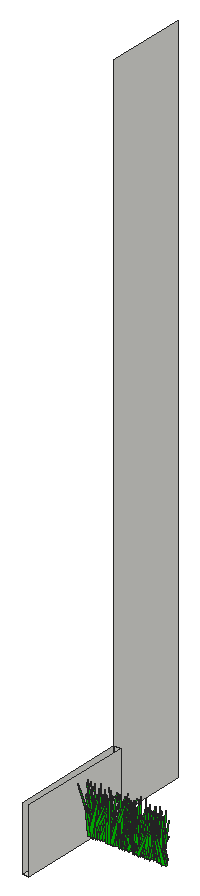
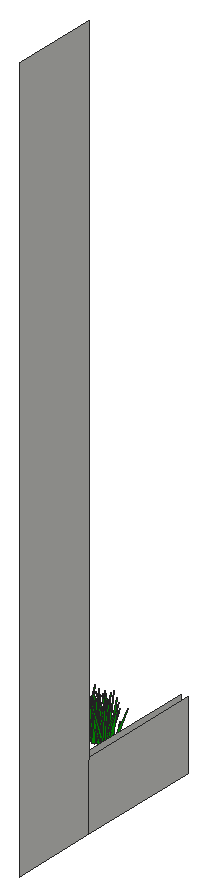
# SketchUp Ruby script. Lengths in inches.
U = 1.inch
M = Sketchup.active_model
def pt(a) = Geom::Point3d.new(a.map { |v| v * U })
def face(e, loops, mat)
  f = e.add_face(loops[0].map { |a| pt(a) })
  loops[1..].each { |l| e.add_face(l.map { |a| pt(a) }).erase! }
  f.material = f.back_material = mat if mat
  f
end
# faces: each face lists its corners as indices into pts; further lists are holes
def faces(e, pts, list, mat = nil) = list.each { |f| face(e, (f[0].is_a?(Array) ? f : [f]).map { |l| l.map { |i| pts[i] } }, mat) }
# xy, xz, yz: faces in a plane at the given z, y or x. An outline is a flat list of corners, or four numbers for a rectangle; further outlines are holes
def ring(l) = l.size == 4 ? [[l[0], l[1]], [l[2], l[1]], [l[2], l[3]], [l[0], l[3]]] : l.each_slice(2).to_a
def flat(e, list, mat, &to3) = list.each { |f| face(e, (f[0].is_a?(Array) ? f : [f]).map { |l| ring(l).map { |u, v| to3.(u, v) } }, mat) }
def xy(e, z, list, mat = nil) = flat(e, list, mat) { |x, y| [x, y, z] }
def xz(e, y, list, mat = nil) = flat(e, list, mat) { |x, z| [x, y, z] }
def yz(e, x, list, mat = nil) = flat(e, list, mat) { |y, z| [x, y, z] }
def lines(e, pts, list) = list.each { |a, b| e.add_line(pt(pts[a]), pt(pts[b])) }
# prism: a flat outline (further loops are holes) pulled along v
def prism(e, loops, v, mat = nil)
  f = face(e, loops, mat); d = Geom::Vector3d.new(v.map { |x| x * U })
  f.pushpull(f.normal.samedirection?(d) ? d.length : -d.length)
end
def box(e, o, s, mat = nil) = prism(e, [[o, [o[0] + s[0], o[1], o[2]], [o[0] + s[0], o[1] + s[1], o[2]], [o[0], o[1] + s[1], o[2]]]], [0, 0, s[2]], mat)
def at(x, y, z, deg = 0) = Geom::Transformation.translation(pt([x, y, z])) * Geom::Transformation.rotation(ORIGIN, Z_AXIS, deg.degrees)
def axes(o, x, y, z) = Geom::Transformation.new([*x, 0, *y, 0, *z, 0, *pt(o).to_a, 1])
def part(name) = M.definitions.add(name)
# library, detail: a bought-in or finely detailed component or shape, given as its bounding box
def library(name, o, s) = part(name).tap { |d| box(d.entities, o, s) }
def detail(e, o, s) = box(e.add_group.entities, o, s)
def put(e, d, t, mat = nil) = e.add_instance(d, t).tap { |i| i.material = mat if mat }
def group(e, t, mat = nil) = e.add_group.tap { |g| g.transformation = t; g.material = mat if mat }.entities
root = M.entities
M.materials.add("[Color G06]").color = [0, 204, 0]
c1 = part("fur_instance\#9")
p = [[0.8125,0,1.79],[0.67,-0.02,1.48],[0,-0.11,0],[0,0.11,0]]
faces(c1.entities,p,[[0,1,2,3]])
xy(root,-6,[[0,8.54,2.44,50.4375]])
xz(root,50.4375,[[0,-6,2.44,17.375]])
yz(root,0,[[8.54,-6,50.4375,17.375],[50.4375,-6,79.8125,242.375]])
yz(root,2.44,[[8.54,-6,50.4375,17.375]])
put(root,c1,axes([12.85,23.35,4.28],[1.6552,-0.74425,1.711],[-5.30221,-0.17956,2.48509],[1.29737,0.21567,7.97338]),"[Color G06]")
put(root,c1,axes([30.55,23.19,4.28],[2.41886,0.55777,0.72324],[3.70499,-0.277,-3.1391],[1.58316,-0.20395,6.24128]),"[Color G06]")
put(root,c1,axes([19.93,23.08,4.28],[3.91287,0.46148,2.2279],[3.1944,-0.58296,1.33945],[-1.72336,-0.03279,7.54123]),"[Color G06]")
put(root,c1,axes([25.93,23.0625,4.28],[5.73991,0.1518,2.08448],[0.76165,-0.80795,2.07407],[-1.5969,0.16027,8.48172]),"[Color G06]")
put(root,c1,axes([28.37,23.59,4.28],[-5.0246,-0.07076,3.70183],[0.48716,0.7269,3.07314],[2.48091,-0.28604,6.89387]),"[Color G06]")
put(root,c1,axes([12.63,23.18,4.28],[-0.11389,0.42663,0.38922],[2.96453,0.00581,1.20582],[-0.79981,-0.03921,4.41401]),"[Color G06]")
put(root,c1,axes([28.8,23.47,4.28],[-3.12756,-0.15217,0.72398],[-0.95592,0.43262,1.2217],[0.71538,-0.0872,4.79764]),"[Color G06]")
put(root,c1,axes([34.63,23.32,4.28],[-0.5319,-0.36164,2.3884],[-2.75252,0.15397,1.30884],[1.30505,0.17735,3.73398]),"[Color G06]")
put(root,c1,axes([33.33,23.2,4.28],[1.33106,0.36919,0.76233],[2.20259,-0.19464,2.23785],[-1.55515,0.04033,3.822]),"[Color G06]")
put(root,c1,axes([28.54,23.35,4.28],[-2.39958,-0.23418,0.91403],[-1.7872,0.31366,-1.24928],[-0.0094,0.14442,4.19532]),"[Color G06]")
put(root,c1,axes([13.41,23.41,4.28],[1.72403,-0.72016,2.8767],[-4.93971,-0.07717,4.39354],[2.4445,0.35197,6.84936]),"[Color G06]")
put(root,c1,axes([30.17,23.48,4.28],[2.8945,0.2824,1.41715],[2.22418,-0.38591,-1.31377],[-0.23073,-0.1774,5.11367]),"[Color G06]")
put(root,c1,axes([25.15,23.2,4.28],[4.85525,0.25985,0.85646],[1.64604,-0.6613,2.20422],[-1.04468,0.16571,7.45353]),"[Color G06]")
put(root,c1,axes([23.65,23.29,4.28],[2.63832,0.09566,1.76868],[0.13664,-0.37516,1.87571],[-1.36103,0.14778,3.61684]),"[Color G06]")
put(root,c1,axes([39.7,23.3,4.28],[-1.60341,0.64726,0.46513],[4.41157,0.19699,2.48074],[-1.47638,-0.11433,6.90756]),"[Color G06]")
put(root,c1,axes([14.0625,23.39,4.28],[2.53929,-0.11197,1.32679],[-1.06003,-0.3452,1.18522],[-0.55601,0.14677,3.79981]),"[Color G06]")
put(root,c1,axes([30.79,23.91,4.28],[4.96251,-0.35133,2.15293],[-1.47007,-0.64737,-4.56652],[-2.50232,-0.31642,6.95237]),"[Color G06]")
put(root,c1,axes([20.78,23.25,4.28],[1.34252,0.72283,0.0164],[5.00506,-0.18035,-2.08662],[1.34888,-0.05024,7.72612]),"[Color G06]")
put(root,c1,axes([29.4375,23.32,4.28],[-1.28557,0.59423,1.27715],[4.16234,0.20409,-1.54961],[1.25078,-0.06842,6.46945]),"[Color G06]")
put(root,c1,axes([32.22,23.53,4.28],[-5.11111,0.1924,0.36372],[1.40056,0.7051,1.11518],[0.03793,-0.10931,7.8334]),"[Color G06]")
put(root,c1,axes([29.77,23.65,4.28],[-1.3987,-0.81448,2.72919],[-5.9965,0.23455,1.17629],[1.22159,0.21879,8.89902]),"[Color G06]")
put(root,c1,axes([20.625,23.68,4.28],[2.09428,-0.78657,0.87313],[-5.32436,-0.24284,3.39616],[1.95198,0.18152,8.32683]),"[Color G06]")
put(root,c1,axes([18.4,23.57,4.28],[2.99741,0.29568,0.585],[2.13228,-0.39259,-1.61022],[0.32024,-0.15348,5.24587]),"[Color G06]")
put(root,c1,axes([24.57,23.56,4.28],[-2.31586,-0.36535,0.62633],[-2.55714,0.28662,-1.91374],[-0.708,0.15984,4.86328]),"[Color G06]")
put(root,c1,axes([33,23.48,4.28],[4.91073,-0.40144,3.20689],[-3.31936,-0.70084,1.27585],[-1.36875,0.25935,8.41144]),"[Color G06]")
put(root,c1,axes([21.69,23.48,4.28],[2.25116,0.46724,2.42365],[3.3843,-0.36695,1.10474],[-1.55026,-0.12258,5.93111]),"[Color G06]")
put(root,c1,axes([15.98,23.37,4.28],[2.98241,0.27292,0.8081],[1.72101,-0.41087,1.75207],[-1.07746,0.09916,5.0354]),"[Color G06]")
put(root,c1,axes([33.29,23.39,4.28],[-0.61548,0.71183,1.08792],[4.98232,0.05576,2.10506],[-1.32848,-0.12066,7.39074]),"[Color G06]")
put(root,c1,axes([28.35,23.79,4.28],[-2.2351,-0.42611,1.57336],[-2.51511,0.3414,2.64062],[2.02982,-0.04618,5.00443]),"[Color G06]")
put(root,c1,axes([38.11,23.43,4.28],[-0.76903,0.72137,2.0022],[5.23961,0.13887,-1.25216],[1.04989,-0.16466,7.71563]),"[Color G06]")
put(root,c1,axes([13.86,23.61,4.28],[2.71632,-0.46654,0.25104],[-3.00104,-0.32551,3.04278],[1.48844,0.1951,5.67683]),"[Color G06]")
put(root,c1,axes([14.85,23.34,4.28],[-3.57418,0.15931,1.87457],[0.45728,0.48323,-2.77015],[1.6338,0.21327,4.87623]),"[Color G06]")
put(root,c1,axes([23,23.73,4.28],[5.38084,0.01238,0.72227],[0.17983,-0.73926,-1.53704],[-0.45725,-0.14506,7.89493]),"[Color G06]")
put(root,c1,axes([16.29,23.63,4.28],[2.30947,0.32228,0.62027],[2.26105,-0.28332,-1.89459],[0.63352,-0.16368,4.50067]),"[Color G06]")
put(root,c1,axes([13.13,23.65,4.28],[1.72877,-0.45008,0.49631],[-2.65707,-0.16626,3.3536],[1.86221,0.1806,4.32429]),"[Color G06]")
put(root,c1,axes([19.2,23.38,4.28],[0.80978,0.69046,0.59357],[4.8898,-0.12068,1.22501],[-0.87466,-0.03542,7.39796]),"[Color G06]")
put(root,c1,axes([18.43,23.79,4.28],[4.45416,-0.00649,0.14759],[-0.01839,-0.59853,-1.78589],[-0.10762,-0.16652,6.41343]),"[Color G06]")
put(root,c1,axes([28.8125,23.49,4.28],[-2.35811,0.38989,1.71965],[2.55865,0.36574,-1.68843],[1.61083,-0.01018,5.19933]),"[Color G06]")
put(root,c1,axes([34.9,23.99,4.28],[3.97939,-0.66126,1.5906],[-4.29861,-0.56838,-3.12205],[-2.26762,-0.08298,8.70959]),"[Color G06]")
put(root,c1,axes([40.57,23.5625,4.28],[-4.2997,-0.26227,1.133],[-2.02384,0.57059,-1.9831],[0.12754,0.21235,6.72796]),"[Color G06]")
put(root,c1,axes([30.6875,23.8,4.28],[1.06399,-0.58128,0.38184],[-3.56039,-0.10703,3.44347],[2.18298,0.10875,5.43011]),"[Color G06]")
put(root,c1,axes([15.04,23.89,4.28],[2.29731,-0.39502,0.33746],[-2.68324,-0.31485,-1.53547],[-0.93594,-0.06694,5.23035]),"[Color G06]")
put(root,c1,axes([26.5,23.68,4.28],[2.69023,-0.58504,0.88466],[-3.7722,-0.28619,3.88244],[1.92943,0.2562,6.35698]),"[Color G06]")
put(root,c1,axes([14.56,23.65,4.28],[-0.73248,0.41655,1.23313],[2.91888,0.05301,1.81602],[-1.04133,-0.14443,4.22295]),"[Color G06]")
put(root,c1,axes([29.15,23.39,4.28],[-5.18337,0.20223,2.51266],[0.67358,0.71057,-3.46575],[2.11562,0.26923,7.25958]),"[Color G06]")
put(root,c1,axes([27.24,24.04,4.28],[4.6175,-0.53623,1.55109],[-3.45439,-0.64944,-2.82084],[-1.98282,-0.11731,8.52646]),"[Color G06]")
put(root,c1,axes([12.73,23.62,4.28],[0.09453,0.44554,0.98091],[3.00479,-0.04752,1.83243],[-1.26901,-0.07932,4.41193]),"[Color G06]")
put(root,c1,axes([24.87,23.93,4.28],[0.85117,-0.81968,1.86534],[-5.90948,-0.14606,-1.34956],[-1.08995,0.1518,8.77372]),"[Color G06]")
put(root,c1,axes([20.83,23.4375,4.28],[2.57475,0.44269,0.089],[2.89983,-0.3322,2.42235],[-1.29337,0.13646,5.60828]),"[Color G06]")
put(root,c1,axes([22.21,23.87,4.28],[-0.28774,-0.41007,0.67375],[-2.84013,0.01906,-1.37689],[-0.88578,0.0721,4.19594]),"[Color G06]")
put(root,c1,axes([35.69,23.99,4.28],[2.57469,-0.15638,1.17423],[-0.73616,-0.35482,-1.82268],[-1.15453,-0.12249,3.78081]),"[Color G06]")
put(root,c1,axes([23.86,24.18,4.28],[5.65623,-0.09199,1.69851],[-0.10142,-0.72878,-3.77975],[-1.31013,-0.34074,7.62561]),"[Color G06]")
put(root,c1,axes([25.31,24.05,4.28],[0.5986,-0.65583,0.86329],[-4.57695,-0.05901,1.93936],[1.22659,0.09986,6.8153]),"[Color G06]")
put(root,c1,axes([38.11,23.78,4.28],[-3.14305,0.62042,0.24122],[4.35481,0.4227,1.85897],[-0.92567,-0.11802,7.92643]),"[Color G06]")
put(root,c1,axes([27.6,23.82,4.28],[-2.3049,0.56321,0.20905],[3.79803,0.2942,2.48689],[-1.3811,-0.13087,6.49009]),"[Color G06]")
put(root,c1,axes([13.4,24.26,4.28],[3.48298,-0.40385,0.45286],[-2.62807,-0.46433,-2.41733],[-1.25403,-0.14857,6.32377]),"[Color G06]")
put(root,c1,axes([25.21,24.04,4.28],[-1.11727,-0.7136,2.77183],[-5.37032,0.10148,-1.83417],[-0.88734,0.28435,7.61066]),"[Color G06]")
put(root,c1,axes([15.2,23.97,4.28],[-0.62082,0.63422,2.42836],[4.26626,-0.03506,3.48816],[-2.2638,-0.24,5.90767]),"[Color G06]")
put(root,c1,axes([18.28,24.29,4.28],[4.03639,-0.52328,0.8731],[-3.64556,-0.56718,-1.40332],[-1.06449,-0.04177,8.11662]),"[Color G06]")
put(root,c1,axes([16.95,24.33,4.28],[-5.99504,0.07316,1.94012],[0.99737,0.78176,3.49768],[0.98266,-0.34711,8.28633]),"[Color G06]")
put(root,c1,axes([17.68,23.76,4.28],[2.25888,0.68942,0.49773],[4.85891,-0.31818,1.37065],[-0.97212,0.01161,8.00742]),"[Color G06]")
put(root,c1,axes([34.36,24.17,4.28],[4.90832,-0.09374,1.53807],[-0.52994,-0.69437,-1.08394],[-1.10912,-0.08307,7.32456]),"[Color G06]")
put(root,c1,axes([23.64,24.22,4.28],[4.85353,0.43456,0.78323],[2.94979,-0.57497,-4.18497],[1.13359,-0.36444,7.53653]),"[Color G06]")
put(root,c1,axes([33.14,23.87,4.28],[0.23123,0.78454,0.57374],[5.58253,-0.02427,-1.21368],[0.79766,-0.05759,8.32782]),"[Color G06]")
put(root,c1,axes([29.89,24.07,4.28],[4.55967,-0.47208,3.92643],[-3.99429,-0.66195,1.21859],[-1.55192,0.3167,8.39983]),"[Color G06]")
put(root,c1,axes([14.77,24.37,4.28],[-5.33008,-0.41735,1.48332],[-2.87754,0.75495,1.30404],[1.2893,-0.04041,9.04261]),"[Color G06]")
put(root,c1,axes([18.85,24.39,4.28],[-1.58104,-0.47887,0.54662],[-3.23778,0.22505,1.72929],[1.20153,-0.02369,5.37923]),"[Color G06]")
put(root,c1,axes([23.72,24.07,4.28],[5.52003,-0.09986,1.70967],[-0.9319,-0.76787,1.56857],[-0.97621,0.16832,8.17002]),"[Color G06]")
put(root,c1,axes([36.8,24.01,4.28],[-4.45501,0.07,2.54988],[0.02623,0.64422,-1.92927],[1.77822,0.16587,6.41673]),"[Color G06]")
put(root,c1,axes([37.35,24.01,4.28],[4.63677,0.19583,1.87939],[1.11358,-0.66023,1.76585],[-1.52098,0.11361,7.02226]),"[Color G06]")
put(root,c1,axes([33.7,24.21,4.28],[3.0211,-0.32881,0.74455],[-2.38533,-0.39204,1.73098],[0.34425,0.16913,5.45997]),"[Color G06]")
put(root,c1,axes([16.6,24.5,4.28],[3.99533,-0.51338,1.99576],[-3.28341,-0.5841,-2.57747],[-2.13463,-0.06245,7.70001]),"[Color G06]")
put(root,c1,axes([24.125,24.5,4.28],[-4.00474,-0.4124,0.52804],[-2.80312,0.54976,1.83568],[1.0069,-0.10976,7.21059]),"[Color G06]")
put(root,c1,axes([36.9,24.42,4.28],[1.18944,-0.40955,0.33369],[-2.83305,-0.16826,-1.16565],[-0.80591,-0.01296,4.59014]),"[Color G06]")
put(root,c1,axes([26.39,24.13,4.28],[3.77808,0.02904,0.15998],[0.18084,-0.51517,1.20264],[-0.14874,0.11128,5.52583]),"[Color G06]")
put(root,c1,axes([27.05,24.39,4.28],[5.23027,-0.06545,2.67994],[-0.15842,-0.76161,-1.44593],[-1.84674,-0.12002,7.71409]),"[Color G06]")
put(root,c1,axes([25.47,24.07,4.28],[-1.56069,0.77606,1.15491],[5.53513,0.19314,1.7994],[-0.96548,-0.14721,8.44916]),"[Color G06]")
put(root,c1,axes([21.08,24.14,4.28],[-5.05472,-0.27366,0.95061],[-2.06113,0.65998,-2.65592],[-0.08739,0.26291,7.65649]),"[Color G06]")
put(root,c1,axes([24.95,24.37,4.28],[2.34007,-0.39721,0.0355],[-2.7999,-0.31993,1.04319],[0.52454,0.0643,5.41002]),"[Color G06]")
put(root,c1,axes([38.57,23.97,4.28],[1.19298,0.83169,0.56408],[5.90274,-0.17237,1.30934],[-0.93395,-0.02706,8.99578]),"[Color G06]")
put(root,c1,axes([28.08,24.36,4.28],[-2.464,-0.53144,0.87564],[-3.78572,0.31502,-1.83279],[-0.73209,0.15967,6.53043]),"[Color G06]")
put(root,c1,axes([24.27,24.5,4.28],[2.93377,-0.03197,1.53084],[0.23777,-0.39273,-1.96011],[-1.02232,-0.18309,3.93716]),"[Color G06]")
put(root,c1,axes([31.17,24.38,4.28],[-1.99382,0.27546,0.31988],[1.88217,0.24828,1.64453],[-0.63682,-0.12864,3.85903]),"[Color G06]")
put(root,c1,axes([28.36,24.49,4.28],[-2.70087,0.06909,1.33588],[0.76625,0.36994,1.26268],[0.6762,-0.14326,3.90493]),"[Color G06]")
put(root,c1,axes([17.76,24.46,4.28],[-2.53271,0.50939,2.26503],[3.90832,0.284,2.42503],[-0.60486,-0.29789,6.18508]),"[Color G06]")
put(root,c1,axes([27.45,24.31,4.28],[1.86772,0.48831,0.49651],[3.41517,-0.23918,-1.67488],[0.84227,-0.11301,5.69018]),"[Color G06]")
put(root,c1,axes([16.41,24.48,4.28],[-2.17137,-0.65597,3.16875],[-4.90501,0.36197,1.09998],[1.60155,0.21924,7.66501]),"[Color G06]")
put(root,c1,axes([29.87,24.09,4.28],[0.51336,0.81685,0.15536],[5.69469,-0.07299,2.05212],[-1.37685,0.00268,8.5456]),"[Color G06]")
put(root,c1,axes([34.97,24.37,4.28],[-3.41166,-0.16628,1.21169],[-1.36717,0.46531,-1.26365],[0.45819,0.15033,5.25154]),"[Color G06]")
put(root,c1,axes([14.28,24.2,4.28],[5.01374,0.31233,0.33916],[2.15317,-0.68782,1.66408],[-0.65742,0.12924,8.03669]),"[Color G06]")
put(root,c1,axes([18.84,24.26,4.28],[-4.37914,0.19277,1.03402],[1.20844,0.60762,-1.58103],[0.96406,0.11399,6.67874]),"[Color G06]")
put(root,c1,axes([29.16,24.34,4.28],[-0.04114,0.59428,1.67097],[4.31126,0.03758,-1.29817],[0.90851,-0.15142,6.23608]),"[Color G06]")
put(root,c1,axes([13.88,24.23,4.28],[-1.16144,0.44519,0.06039],[3.03497,0.1558,-1.55586],[0.9915,0.04459,4.83321]),"[Color G06]")
put(root,c1,axes([16.01,24.12,4.28],[1.60528,0.71227,0.01705],[4.91274,-0.21575,2.18547],[-1.39829,0.05968,7.69797]),"[Color G06]")
put(root,c1,axes([30.5625,24.43,4.28],[-4.03167,0.41913,0.43889],[2.99067,0.54461,1.62187],[-0.41983,-0.14542,7.33879]),"[Color G06]")
put(root,c1,axes([19.39,24.63,4.28],[1.73605,-0.63922,2.52921],[-4.45285,-0.31008,-2.17531],[-2.01228,0.13469,6.99564]),"[Color G06]")
put(root,c1,axes([18.45,24.46,4.28],[1.66352,0.31797,0.4858],[2.24642,-0.21162,-1.27089],[0.50883,-0.10526,4.02257]),"[Color G06]")
put(root,c1,axes([34.53,24.7,4.28],[4.16379,0.23735,5.12817],[2.6616,-0.68751,-1.17195],[-2.75427,-0.30557,6.62003]),"[Color G06]")
put(root,c1,axes([29.79,24.49,4.28],[4.58622,-0.36641,1.31176],[-2.76799,-0.61579,1.8579],[-0.11375,0.2116,7.67817]),"[Color G06]")
put(root,c1,axes([24.64,24.54,4.28],[4.35925,-0.42263,2.27991],[-3.30356,-0.60766,1.16969],[-0.77398,0.21333,7.84844]),"[Color G06]")
put(root,c1,axes([35.79,24.63,4.28],[2.60086,-0.48243,0.46474],[-3.34574,-0.33337,2.07153],[0.93373,0.14927,6.12821]),"[Color G06]")
put(root,c1,axes([34.88,24.42,4.28],[-5.10141,0.07727,2.2531],[0.1651,0.72152,-2.00744],[1.59762,0.17216,7.40188]),"[Color G06]")
put(root,c1,axes([28.99,24.84,4.28],[4.57152,-0.1299,0.61615],[-0.74377,-0.60623,-2.35503],[-0.69606,-0.20534,6.56314]),"[Color G06]")
put(root,c1,axes([34.86,24.33,4.28],[3.34015,0.5562,0.42724],[3.85535,-0.46169,1.71858],[-1.06191,0.0733,7.58325]),"[Color G06]")
put(root,c1,axes([23.71,24.59,4.28],[1.04205,0.43088,2.51292],[3.11835,-0.22632,1.56929],[-1.62808,-0.15769,4.61414]),"[Color G06]")
put(root,c1,axes([24.45,24.96,4.28],[-3.0588,-0.63316,0.34063],[-4.33921,0.41802,2.22161],[1.35642,-0.09054,7.87505]),"[Color G06]")
put(root,c1,axes([19.25,24.33,4.28],[5.53598,0.35845,1.15639],[2.29329,-0.76003,2.53958],[-1.39535,0.17299,8.76174]),"[Color G06]")
put(root,c1,axes([36.08,24.62,4.28],[-4.95357,0.41244,1.03628],[3.03171,0.68297,1.1454],[0.19432,-0.14154,8.5464]),"[Color G06]")
put(root,c1,axes([17.77,24.66,4.28],[-2.67563,0.63215,2.45607],[4.81176,0.33301,1.86324],[-0.31319,-0.2843,7.64361]),"[Color G06]")
put(root,c1,axes([23.14,24.78,4.28],[1.59433,-0.60923,1.33971],[-4.35867,-0.18471,1.93754],[0.94513,0.17588,6.67542]),"[Color G06]")
put(root,c1,axes([18.27,24.68,4.28],[2.93803,0.36191,0.03875],[2.44797,-0.38458,-1.98815],[0.86242,-0.14128,5.51133]),"[Color G06]")
put(root,c1,axes([18.38,24.66,4.28],[-2.10762,0.37801,0.62443],[2.70358,0.27393,1.33404],[-0.46224,-0.12137,4.95554]),"[Color G06]")
put(root,c1,axes([33.61,24.54,4.28],[4.10155,0.40455,2.47492],[2.62036,-0.61643,1.87476],[-2.07181,0.02124,7.27074]),"[Color G06]")
put(root,c1,axes([37.2,24.24,4.28],[-5.06234,0.48915,0.77232],[2.81137,0.63029,-4.69428],[2.16054,0.32596,7.91797]),"[Color G06]")
put(root,c1,axes([21.52,24.89,4.28],[-6.04082,-0.06233,1.58493],[-0.26157,0.84387,1.5856],[1.1207,-0.13903,8.9132]),"[Color G06]")
put(root,c1,axes([26.17,24.95,4.28],[-1.97717,-0.37784,0.01658],[-2.64471,0.26952,1.07902],[0.58959,-0.05812,4.89571]),"[Color G06]")
put(root,c1,axes([29.14,24.86,4.28],[-1.55553,-0.47492,0.72604],[-3.40442,0.20181,-1.12871],[-0.49503,0.10447,5.48093]),"[Color G06]")
put(root,c1,axes([21.89,24.98,4.28],[5.48863,0.17212,1.32019],[1.47514,-0.71372,-3.01005],[-0.35739,-0.30259,7.85076]),"[Color G06]")
put(root,c1,axes([28.8125,24.61,4.28],[2.41467,0.11269,1.67204],[0.17245,-0.33656,2.04936],[-1.36927,0.15633,3.20672]),"[Color G06]")
put(root,c1,axes([26.41,25.01,4.28],[-1.57556,-0.45631,0.4597],[-3.15034,0.22322,1.33503],[0.93703,-0.01677,5.26135]),"[Color G06]")
put(root,c1,axes([24.33,24.65,4.28],[-3.21397,0.08301,0.7555],[0.38502,0.42815,-1.7455],[0.67946,0.15005,4.56274]),"[Color G06]")
put(root,c1,axes([25.15,24.98,4.28],[3.72994,-0.06378,1.441],[-0.16223,-0.51699,-1.69048],[-1.05473,-0.14602,5.35598]),"[Color G06]")
put(root,c1,axes([19.72,24.89,4.28],[-1.43027,-0.56381,1.29677],[-3.9983,0.15587,-2.06559],[-1.05541,0.17355,6.06787]),"[Color G06]")
put(root,c1,axes([26.07,24.67,4.28],[-1.99806,0.39808,0.80436],[2.68018,0.28774,-1.48712],[1.1206,0.02158,4.99099]),"[Color G06]")
put(root,c1,axes([22.02,24.97,4.28],[-1.52671,-0.57825,2.2682],[-4.18052,0.26139,1.36944],[1.42208,0.1476,6.46084]),"[Color G06]")
put(root,c1,axes([33.17,24.79,4.28],[5.66482,-0.04197,2.1604],[-0.49298,-0.80709,1.08627],[-1.39177,0.11505,8.40855]),"[Color G06]")
put(root,c1,axes([34.01,24.79,4.28],[5.29304,-0.32996,1.39533],[-2.53789,-0.70543,2.34159],[-0.17294,0.25317,8.34298]),"[Color G06]")
put(root,c1,axes([29.46,24.75,4.28],[0.42581,0.41367,0.72142],[2.676,-0.08313,1.94776],[-1.36838,-0.03384,4.03351]),"[Color G06]")
put(root,c1,axes([21.59,24.97,4.28],[4.72239,0.41083,2.38227],[3.29063,-0.6408,-1.87632],[-0.62629,-0.26912,8.1045]),"[Color G06]")
put(root,c1,axes([35.99,24.98,4.28],[1.61057,-0.34728,0.20315],[-2.41578,-0.2116,1.22892],[0.62026,0.07762,4.25889]),"[Color G06]")
put(root,c1,axes([36.64,24.81,4.28],[-4.80183,-0.26915,1.78913],[-2.1987,0.64873,-1.97064],[0.56932,0.2353,7.47951]),"[Color G06]")
put(root,c1,axes([31.47,24.82,4.28],[4.45919,0.01082,2.02166],[-0.16012,-0.64006,1.18226],[-1.34539,0.11202,6.55991]),"[Color G06]")
put(root,c1,axes([31.24,24.89,4.28],[-0.41775,0.42168,1.3297],[3.07993,0.02797,1.14244],[-0.67083,-0.13417,4.41714]),"[Color G06]")
put(root,c1,axes([12.54,25.24,4.28],[3.57657,-0.44084,0.45557],[-2.92937,-0.48261,-2.27645],[-1.22725,-0.13278,6.7614]),"[Color G06]")
put(root,c1,axes([29.93,24.98,4.28],[-2.30406,-0.41171,0.20245],[-2.72168,0.28621,-2.32686],[-1.15238,0.14719,5.09078]),"[Color G06]")
put(root,c1,axes([17.3125,25.05,4.28],[-1.51635,-0.47286,0.34803],[-3.20576,0.18714,-1.991],[-1.12976,0.10365,5.18248]),"[Color G06]")
put(root,c1,axes([26.6,24.63,4.28],[-4.98106,0.42569,1.35265],[2.65896,0.68501,-2.89325],[1.75168,0.17068,8.23818]),"[Color G06]")
put(root,c1,axes([25.8,25.21,4.28],[1.33187,-0.60705,0.70882],[-4.07246,-0.19711,-2.29943],[-1.60975,-0.00359,6.40371]),"[Color G06]")
put(root,c1,axes([28.48,24.91,4.28],[1.08394,0.37988,0.71804],[2.69006,-0.12799,-1.29275],[0.64469,-0.10466,4.18694]),"[Color G06]")
put(root,c1,axes([25.95,24.89,4.28],[2.53573,-0.28258,1.20338],[-2.15676,-0.29964,2.06866],[0.32135,0.21875,4.38823]),"[Color G06]")
put(root,c1,axes([18.58,25.09,4.28],[0.06622,-0.48772,1.42164],[-3.4933,0.0268,1.41957],[0.96679,0.13023,5.03191]),"[Color G06]")
put(root,c1,axes([27.84,24.6875,4.28],[4.1698,0.37673,2.02947],[1.94669,-0.58129,3.46129],[-2.3137,0.18988,6.56979]),"[Color G06]")
put(root,c1,axes([14.18,24.85,4.28],[-3.42714,-0.26262,3.87406],[-2.70241,0.52126,-1.28091],[1.72126,0.2955,5.70247]),"[Color G06]")
put(root,c1,axes([21.07,24.73,4.28],[4.07533,0.39825,0.17037],[2.73721,-0.55176,1.90753],[-0.82289,0.13697,7.18886]),"[Color G06]")
put(root,c1,axes([21.73,24.87,4.28],[-1.19378,0.58193,0.33575],[3.99434,0.14929,1.99962],[-1.22927,-0.08003,6.17142]),"[Color G06]")
put(root,c1,axes([35.34,25.04,4.28],[1.18042,-0.56901,2.17399],[-4.06452,-0.07274,2.74258],[1.49868,0.25089,5.72572]),"[Color G06]")
put(root,c1,axes([18.99,25.1,4.28],[4.02334,0.15813,1.0364],[1.25032,-0.55484,-1.11756],[-0.45105,-0.12754,6.14667]),"[Color G06]")
put(root,c1,axes([34.52,24.93,4.28],[0.77918,0.47376,1.20207],[3.27754,-0.13885,1.54088],[-1.20304,-0.07144,4.97648]),"[Color G06]")
put(root,c1,axes([21.89,24.98,4.28],[-2.93237,0.42572,0.08637],[2.97746,0.39617,1.4839],[-0.67721,-0.10157,6.15024]),"[Color G06]")
put(root,c1,axes([16.82,24.88,4.28],[3.70362,0.18066,1.74995],[0.79135,-0.51491,2.36539],[-1.55665,0.16806,5.36601]),"[Color G06]")
put(root,c1,axes([29.26,25,4.28],[-3.26366,-0.16088,2.24405],[-1.57344,0.46252,-1.30257],[1.0534,0.19243,5.00692]),"[Color G06]")
put(root,c1,axes([34.36,25.38,4.28],[-4.6761,-0.03936,2.52711],[0.38712,0.64307,2.75072],[1.66997,-0.25929,6.43851]),"[Color G06]")
put(root,c1,axes([22.9,24.95,4.28],[-5.01813,-0.36412,0.55354],[-2.4318,0.59586,-4.21786],[-1.02074,0.37051,7.32732]),"[Color G06]")
put(root,c1,axes([15.91,25.1,4.28],[3.02482,0.46385,1.09309],[3.40108,-0.40419,-1.32022],[0.17967,-0.15794,6.58868]),"[Color G06]")
put(root,c1,axes([22.39,25.21,4.28],[1.989,-0.35656,0.46445],[-2.53703,-0.26173,1.18774],[0.44518,0.10151,4.6937]),"[Color G06]")
put(root,c1,axes([34.0625,25.22,4.28],[4.48188,0.29367,2.04706],[2.36061,-0.62594,-1.22966],[-0.85937,-0.18783,7.29826]),"[Color G06]")
put(root,c1,axes([22.55,25.12,4.28],[-1.61593,0.42398,0.48616],[2.92727,0.19966,1.73187],[-0.88404,-0.11389,4.84599]),"[Color G06]")
put(root,c1,axes([19.16,25.2,4.28],[1.95777,-0.34842,0.29972],[-2.18686,-0.22007,2.52018],[1.22516,0.16396,4.01945]),"[Color G06]")
put(root,c1,axes([37.64,25.5625,4.28],[-2.55952,-0.65502,1.74272],[-4.00254,0.38988,3.70285],[2.72108,-0.04264,7.08591]),"[Color G06]")
put(root,c1,axes([22.53,25.29,4.28],[4.22134,0.50177,1.13181],[3.62811,-0.54217,-2.615],[0.59867,-0.25241,7.86698]),"[Color G06]")
put(root,c1,axes([12.72,25.33,4.28],[-2.99876,-0.66898,0.92218],[-4.49042,0.3474,-3.66656],[-1.79791,0.24814,7.61936]),"[Color G06]")
put(root,c1,axes([23.35,25.37,4.28],[1.41882,-0.70047,3.09517],[-5.19245,-0.2627,-1.51279],[-1.60017,0.23136,7.6533]),"[Color G06]")
put(root,c1,axes([13.5,25.0625,4.28],[-0.0761,0.84383,1.29124],[5.88367,-0.02256,2.46816],[-1.65757,-0.11882,8.70162]),"[Color G06]")
put(root,c1,axes([24.24,25.13,4.28],[2.07257,0.31355,0.14223],[2.17111,-0.28331,1.07709],[-0.59284,0.05866,4.44175]),"[Color G06]")
put(root,c1,axes([26.25,25.05,4.28],[-6.05862,0.15584,0.0292],[1.06583,0.81,-2.6226],[0.33674,0.24016,8.82644]),"[Color G06]")
put(root,c1,axes([39.28,25.52,4.28],[-4.34807,-0.0869,1.07712],[-0.40453,0.59348,1.85254],[0.86261,-0.15971,6.29811]),"[Color G06]")
put(root,c1,axes([14.99,25.41,4.28],[-3.13472,-0.50677,0.47989],[-3.41477,0.38677,-2.90699],[-1.28439,0.20854,6.55751]),"[Color G06]")
put(root,c1,axes([15.22,25.73,4.28],[3.88477,-0.36855,1.18634],[-2.02512,-0.51057,-3.408],[-1.87464,-0.21218,6.14]),"[Color G06]")
put(root,c1,axes([12.28,25.15,4.28],[3.52148,0.63854,1.2445],[4.48211,-0.5045,1.40541],[-1.25395,-0.01005,8.51841]),"[Color G06]")
put(root,c1,axes([35.25,25.67,4.28],[-4.45241,-0.52903,2.13706],[-3.4301,0.64941,2.5042],[2.16145,-0.05918,8.37621]),"[Color G06]")
put(root,c1,axes([36.1,25.52,4.28],[4.30378,0.1005,1.84521],[0.992,-0.6032,-1.3944],[-1.02936,-0.16113,6.37108]),"[Color G06]")
put(root,c1,axes([20.98,25.08,4.28],[-4.93582,0.48938,0.1127],[3.38939,0.66914,-2.2017],[0.91332,0.16152,8.77973]),"[Color G06]")
put(root,c1,axes([13.39,25.26,4.28],[-0.61586,0.77985,1.4101],[5.39921,0.0401,2.71974],[-1.73634,-0.15191,7.95697]),"[Color G06]")
put(root,c1,axes([18.46,25.53,4.28],[2.12554,-0.5577,2.47529],[-4.07149,-0.34494,-1.1182],[-1.47002,0.149,6.67611]),"[Color G06]")
put(root,c1,axes([37.05,25.51,4.28],[0.41775,-0.44076,1.18576],[-2.9313,-0.00208,2.21789],[1.42403,0.12501,4.21758]),"[Color G06]")
put(root,c1,axes([30.06,25.74,4.28],[-5.37249,-0.37238,0.5564],[-2.5104,0.73307,2.21433],[0.98377,-0.16297,8.68911]),"[Color G06]")
put(root,c1,axes([20.88,25.7,4.28],[1.25919,-0.51582,0.02649],[-3.60093,-0.17152,-1.32786],[-0.84663,-0.03765,5.68712]),"[Color G06]")
put(root,c1,axes([38.17,25.22,4.28],[4.6278,0.4568,1.96123],[3.00203,-0.66824,2.05631],[-1.85497,0.05817,8.22079]),"[Color G06]")
put(root,c1,axes([38.6875,25.26,4.28],[-5.83982,-0.01808,2.18974],[-0.53283,0.80569,-2.40993],[1.37095,0.23612,8.39097]),"[Color G06]")
put(root,c1,axes([35.51,25.61,4.28],[4.03571,-0.47965,2.68071],[-3.36594,-0.61239,-1.26812],[-1.9285,0.06509,7.82314]),"[Color G06]")
put(root,c1,axes([35.72,25.62,4.28],[0.30936,-0.39313,0.38618],[-2.72432,-0.0512,-1.11231],[-0.77005,0.02319,4.09032]),"[Color G06]")
put(root,c1,axes([23.7,25.37,4.28],[3.46617,0.71103,0.92049],[5.05353,-0.45365,-2.25258],[0.91691,-0.18761,8.93529]),"[Color G06]")
put(root,c1,axes([15.81,25.33,4.28],[-4.34968,-0.23337,0.53447],[-1.65453,0.53868,-3.05865],[-0.43718,0.28321,6.25802]),"[Color G06]")
put(root,c1,axes([27.29,25.19,4.28],[-3.68643,0.4014,0.105],[2.6719,0.48279,-2.48058],[1.07336,0.1768,6.53545]),"[Color G06]")
put(root,c1,axes([38.82,25.41,4.28],[-5.26145,-0.20877,0.21992],[-1.47649,0.70234,-2.31428],[-0.28821,0.21314,7.84139]),"[Color G06]")
put(root,c1,axes([14.78,25.47,4.28],[4.6261,-0.20677,0.44238],[-1.51086,-0.62675,1.63945],[0.06086,0.15821,7.07303]),"[Color G06]")
put(root,c1,axes([39.11,25.59,4.28],[-3.94157,0.4105,1.27656],[3.05662,0.51184,2.17391],[-0.22967,-0.23302,7.02392]),"[Color G06]")
put(root,c1,axes([13.39,25.16,4.28],[-2.73784,0.61312,0.288],[3.82614,0.34722,-3.66878],[2.17491,0.16097,6.81671]),"[Color G06]")
put(root,c1,axes([38.52,25.4,4.28],[0.26604,0.4534,0.49145],[3.13647,-0.04835,1.33109],[-0.91794,-0.03378,4.69056]),"[Color G06]")
put(root,c1,axes([29.85,25.33,4.28],[5.49196,-0.08483,4.47855],[-1.55903,-0.81664,2.49356],[-2.63035,0.30691,7.87288]),"[Color G06]")
put(root,c1,axes([29.85,25.54,4.28],[3.02423,0.63211,1.65014],[4.65874,-0.39921,-1.50506],[0.25253,-0.20538,8.00407]),"[Color G06]")
put(root,c1,axes([23.17,25.65,4.28],[-1.47843,-0.62718,3.25721],[-4.75546,0.27403,1.23977],[1.53754,0.24447,6.96646]),"[Color G06]")
put(root,c1,axes([31.16,25.43,4.28],[-2.03943,0.81254,1.39654],[5.8156,0.30014,-1.08949],[1.0024,-0.08816,9.16221]),"[Color G06]")
put(root,c1,axes([34.21,25.65,4.28],[2.53461,-0.36792,1.70101],[-2.86598,-0.30841,1.87611],[0.20745,0.2345,5.13622]),"[Color G06]")
put(root,c1,axes([21.67,25.6,4.28],[5.84548,-0.10965,1.73863],[-1.00774,-0.81125,1.6908],[-0.97777,0.18058,8.65151]),"[Color G06]")
put(root,c1,axes([27.47,25.625,4.28],[5.27069,-0.14972,2.74052],[-1.43854,-0.75472,1.44345],[-1.56387,0.18963,7.90857]),"[Color G06]")
put(root,c1,axes([14.85,25.67,4.28],[5.09072,-0.23389,0.23241],[-1.6628,-0.68672,1.96915],[0.26931,0.18115,7.76499]),"[Color G06]")
put(root,c1,axes([27.46,25.61,4.28],[0.46256,0.74728,1.31156],[5.10282,-0.01781,-2.85416],[1.85721,-0.13718,7.51535]),"[Color G06]")
put(root,c1,axes([27.83,25.65,4.28],[4.41459,-0.35251,1.75638],[-2.78414,-0.54191,3.13718],[0.1416,0.33487,6.9257]),"[Color G06]")
put(root,c1,axes([35.94,25.6,4.28],[-0.27542,0.62461,0.7478],[4.28041,0.05814,-2.05687],[1.41137,-0.05443,6.38402]),"[Color G06]")
put(root,c1,axes([26.32,25.7,4.28],[3.05182,0.34929,1.71953],[2.31935,-0.45474,1.41616],[-1.48948,0.00757,5.72833]),"[Color G06]")
put(root,c1,axes([13.83,25.63,4.28],[-5.18536,0.22144,3.81675],[0.8196,0.78702,-2.75809],[2.89337,0.17392,7.62148]),"[Color G06]")
put(root,c1,axes([23.45,25.61,4.28],[1.50444,0.71298,0.88159],[4.74,-0.22532,2.8653],[-2.00576,0.0023,7.4325]),"[Color G06]")
